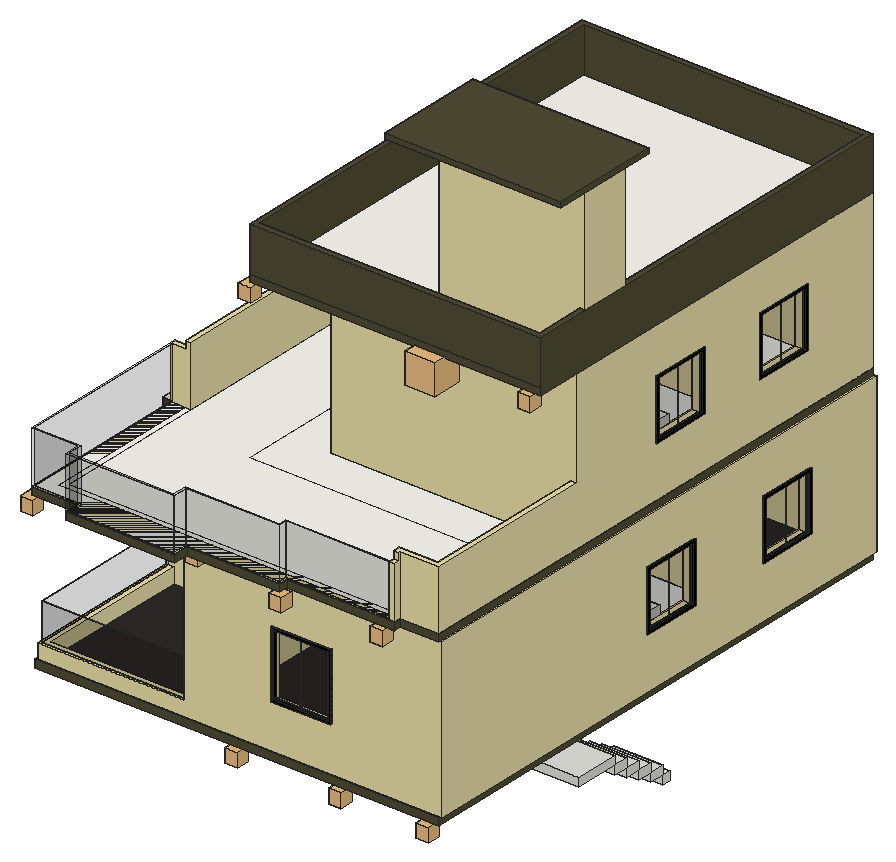
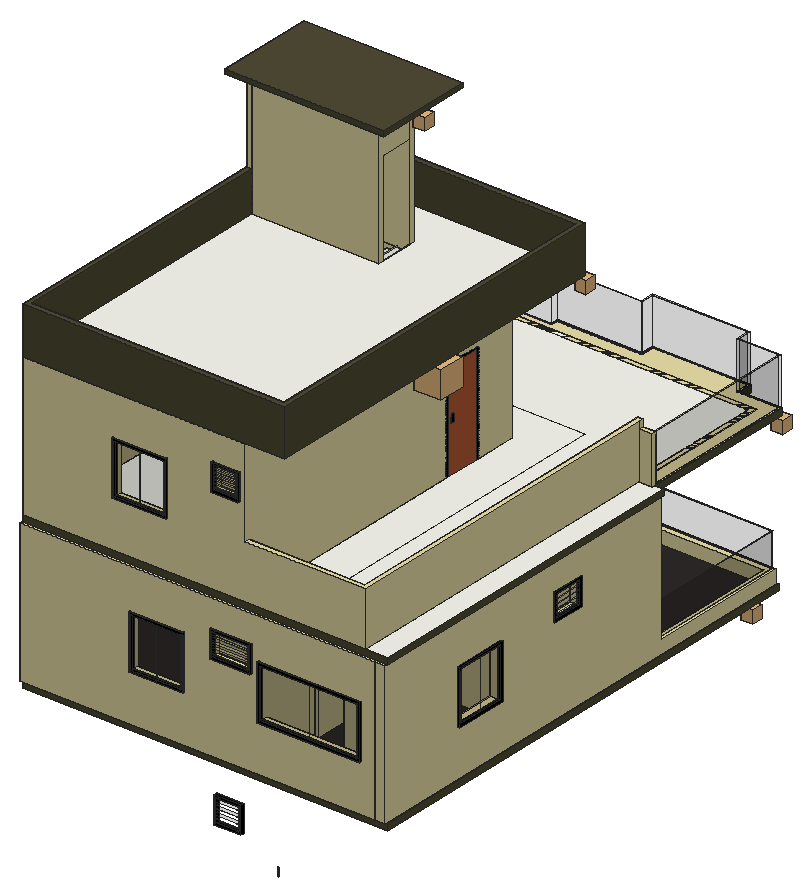
# SketchUp Ruby script. Lengths in inches.
U = 1.inch
M = Sketchup.active_model
def pt(a) = Geom::Point3d.new(a.map { |v| v * U })
def face(e, loops, mat)
  f = e.add_face(loops[0].map { |a| pt(a) })
  loops[1..].each { |l| e.add_face(l.map { |a| pt(a) }).erase! }
  f.material = f.back_material = mat if mat
  f
end
# faces: each face lists its corners as indices into pts; further lists are holes
def faces(e, pts, list, mat = nil) = list.each { |f| face(e, (f[0].is_a?(Array) ? f : [f]).map { |l| l.map { |i| pts[i] } }, mat) }
# xy, xz, yz: faces in a plane at the given z, y or x. An outline is a flat list of corners, or four numbers for a rectangle; further outlines are holes
def ring(l) = l.size == 4 ? [[l[0], l[1]], [l[2], l[1]], [l[2], l[3]], [l[0], l[3]]] : l.each_slice(2).to_a
def flat(e, list, mat, &to3) = list.each { |f| face(e, (f[0].is_a?(Array) ? f : [f]).map { |l| ring(l).map { |u, v| to3.(u, v) } }, mat) }
def xy(e, z, list, mat = nil) = flat(e, list, mat) { |x, y| [x, y, z] }
def xz(e, y, list, mat = nil) = flat(e, list, mat) { |x, z| [x, y, z] }
def yz(e, x, list, mat = nil) = flat(e, list, mat) { |y, z| [x, y, z] }
def lines(e, pts, list) = list.each { |a, b| e.add_line(pt(pts[a]), pt(pts[b])) }
# prism: a flat outline (further loops are holes) pulled along v
def prism(e, loops, v, mat = nil)
  f = face(e, loops, mat); d = Geom::Vector3d.new(v.map { |x| x * U })
  f.pushpull(f.normal.samedirection?(d) ? d.length : -d.length)
end
def box(e, o, s, mat = nil) = prism(e, [[o, [o[0] + s[0], o[1], o[2]], [o[0] + s[0], o[1] + s[1], o[2]], [o[0], o[1] + s[1], o[2]]]], [0, 0, s[2]], mat)
def at(x, y, z, deg = 0) = Geom::Transformation.translation(pt([x, y, z])) * Geom::Transformation.rotation(ORIGIN, Z_AXIS, deg.degrees)
def axes(o, x, y, z) = Geom::Transformation.new([*x, 0, *y, 0, *z, 0, *pt(o).to_a, 1])
def part(name) = M.definitions.add(name)
# library, detail: a bought-in or finely detailed component or shape, given as its bounding box
def library(name, o, s) = part(name).tap { |d| box(d.entities, o, s) }
def detail(e, o, s) = box(e.add_group.entities, o, s)
def put(e, d, t, mat = nil) = e.add_instance(d, t).tap { |i| i.material = mat if mat }
def group(e, t, mat = nil) = e.add_group.tap { |g| g.transformation = t; g.material = mat if mat }.entities
root = M.entities
M.materials.add("BLack FLOOR").color = [47, 42, 42]
M.materials.add("METAL").color = [0, 0, 0]
M.materials.add("WALL PAINT").color = [235, 224, 170]
M.materials.add("WALL PAINT\#1").color = [80, 76, 53]
M.materials.add("WHITE FLOOR").color = [250, 250, 243]
M.materials.add("glass").color = [0, 0, 0]
M.materials["glass"].alpha = 0.1
M.materials.add("wood").color = [181, 91, 54]
c1 = part("Component\#8")
box(c1.entities,[4.875,0,0],[7.125,36,7])
c2 = part("Stair tread")
box(c2.entities,[0,0,0],[12,39.4375,7])
c3 = library("Omni Light\#4",[-12,-12,-12],[24,24,24])
c4 = part("Stair landing \#4")
box(c4.entities,[-1.5,0,0],[36,39.4375,7])
c5 = part("Stair tread \#5")
box(c5.entities,[0,0,0],[12,39.4375,7])
c6 = library("Omni Light",[-12,-12,-12],[24,24,24])
c7 = library("Spot Light\#4",[-5.1,-5.1,-11.05],[10.2,10.2,11.05])
c8 = library("Spot Light\#5",[-5.1,-5.1,-11.05],[10.2,10.2,11.05])
c9 = library("Spot Light\#6",[-5.1,-5.1,-11.05],[10.2,10.2,11.05])
c10 = library("Spot Light\#7",[-5.1,-5.1,-11.05],[10.2,10.2,11.05])
c11 = library("Spot Light\#3",[-5.1,-5.1,-11.05],[10.2,10.2,11.05])
c12 = part("Stair tread \#1")
box(c12.entities,[-3.4375,0,0],[12,39.4375,7])
c13 = part("Stair landing")
box(c13.entities,[0,0,0],[39.4375,36,7])
c14 = part("Stair landing \#1")
box(c14.entities,[-1.5,0,0],[36,39.4375,7])
c15 = part("Stair tread \#3")
box(c15.entities,[-3.4375,0,0],[12,34.5,7])
c16 = part("Group173\#1")
p = [[0,0,0],[0,0,-9.21],[-2.27,0,-9.21],[14.78,-15.03,0],[-14.78,-15.03,0],[14.78,15.03,0],
  [14.78,0,0],[-14.78,15.03,0],[2.27,0,-9.21],[-14.78,0,0],[0,0,-14.91]]
lines(c16.entities,p,[[0,1],[1,2],[3,4],[5,6],[7,5],[1,8],[9,0],[0,6],[8,10],[4,9],[6,3],[2,10],
  [9,7]])
c17 = part("Rectangle Light")
put(c17.entities,c16,at(0,0,0))
c18 = library("Omni Light\#5",[-12,-12,-12],[24,24,24])
c19 = library("Omni Light\#1",[-12,-12,-12],[24,24,24])
c20 = library("Spot Light",[-5.1,-5.1,-11.05],[10.2,10.2,11.05])
c21 = library("Spot Light\#1",[-5.1,-5.1,-11.05],[10.2,10.2,11.05])
c22 = library("Spot Light\#2",[-5.1,-5.1,-11.05],[10.2,10.2,11.05])
c23 = library("Spot Light\#8",[-5.1,-5.1,-11.05],[10.2,10.2,11.05])
c24 = part("Stair tread \#2")
box(c24.entities,[0,0,0],[12,36,7])
c25 = part("Stair landing \#2")
box(c25.entities,[0,0,0],[36,36,7])
c26 = part("Stair landing \#3")
box(c26.entities,[-22.1875,0,0],[34.1875,36,7])
c27 = part("Stair tread \#4")
box(c27.entities,[-22.1875,0,0],[34.1875,12,7])
c28 = library("Omni Light\#2",[-12,-12,-12],[24,24,24])
c29 = library("Omni Light\#3",[-12,-12,-12],[24,24,24])
c30 = library("Spot Light\#9",[-5.1,-5.1,-11.05],[10.2,10.2,11.05])
c31 = library("Spot Light\#10",[-5.1,-5.1,-11.05],[10.2,10.2,11.05])
c32 = library("Spot Light\#11",[-5.1,-5.1,-11.05],[10.2,10.2,11.05])
put(root,c1,at(288,397.9,54.4375,-90))
g1 = group(root,at(112.46,576,55.32),"METAL")
box(g1,[0,0,0],[1.1,0.5,6.84])
put(root,c2,at(284.5625,385.9,61.4375,-90))
put(root,c2,at(284.5625,373.9,68.4375,-90))
put(root,c2,at(284.5625,361.9,75.4375,-90))
put(root,c3,at(252,402,93.375))
put(root,c2,at(284.5625,349.9,82.4375,-90))
g2 = group(root,at(138,585,83.4375))
prism(g2,[[[24,-1.5,24],[0,-1.5,24],[0,-1.5,0],[24,-1.5,0]],[[22,-1.5,22],[22,-1.5,2],[2,-1.5,2],[2,-1.5,22]]],[0,3,0],"METAL")
g3 = group(root,at(140,586.5,85.4375))
box(g3,[0,0,0],[20,0.2,3.53],"glass")
put(root,c4,at(284.5625,336.4,89.4375,-90))
g4 = group(root,at(140,586.5,90.93))
box(g4,[0,0,0],[20,0.2,3.53],"glass")
g5 = group(root,at(140,586.5,96.42))
box(g5,[0,0,0],[20,0.2,3.53],"glass")
g6 = group(root,at(224.5625,301.9,89.4375))
put(g6,c5,at(0,0,35))
put(g6,c2,at(48,0,7))
put(g6,c2,at(36,0,14))
put(g6,c2,at(12,0,28))
put(g6,c2,at(24,0,21))
g7 = group(root,at(140,586.5,101.91))
box(g7,[0,0,0],[20,0.2,3.53],"glass")
put(root,c6,at(106.39,205.09,117.1875))
put(root,c7,at(93.68,171.67,131.43))
put(root,c8,at(171,150,131.43))
put(root,c9,at(253.9375,150,131.43))
put(root,c10,at(324.18,150,131.43))
put(root,c11,at(10.5,179.06,132.58))
g8 = group(root,at(32,150,131.4375),"WALL PAINT\#1")
xy(g8,0,[[[-23,0,301,435],[192.5625,151.1875,292,271.5]]],"WALL PAINT\#1")
xy(g8,6,[[[-23,0,301,435],[192.5625,151.1875,292,271.5]]],"BLack FLOOR")
xz(g8,0,[[-23,0,301,6]],"WALL PAINT\#1")
xz(g8,151.1875,[[192.5625,0,292,6]],"WALL PAINT\#1")
xz(g8,271.5,[[192.5625,0,292,6]],"WALL PAINT\#1")
xz(g8,435,[[-23,0,301,6]],"WALL PAINT\#1")
yz(g8,-23,[[0,0,435,6]],"WALL PAINT\#1")
yz(g8,192.5625,[[151.1875,0,271.5,6]],"WALL PAINT\#1")
yz(g8,292,[[151.1875,0,271.5,6]],"WALL PAINT\#1")
yz(g8,301,[[0,0,435,6]],"WALL PAINT\#1")
g9 = group(root,at(9,150,137.4375))
put(g9,c12,at(256.5,230.5,21))
put(g9,c12,at(277.0625,215.0625,49,-90))
put(g9,c12,at(232.5,230.5,7))
put(g9,c12,at(244.5,230.5,14))
put(g9,c13,at(277.0625,230.5,35))
put(g9,c12,at(277.0625,191.0625,63,-90))
put(g9,c12,at(277.0625,179.0625,70,-90))
put(g9,c12,at(220.5,230.5,0))
put(g9,c12,at(268.5,230.5,28))
put(g9,c14,at(277.0625,169,77,-90))
put(g9,c12,at(277.0625,227.0625,42,-90))
put(g9,c15,at(268.5,136,84))
put(g9,c12,at(277.0625,203.0625,56,-90))
put(g9,c15,at(256.5,136,91))
put(g9,c15,at(244.5,136,98))
put(g9,c15,at(232.5,136,105))
put(g9,c15,at(220.5,136,112))
put(g9,c15,at(208.5,136,119))
put(g9,c17,axes([157,118.76,110.97],[-0.60781,0.79408,0],[0,0,-1],[0.79408,0.60781,0]))
put(g9,c18,at(205.65,130.5,40.02))
g10 = group(g9,at(325.4375,324.24,44))
box(g10,[-0.31,0,0],[0.31,22,44],"glass")
g11 = group(g9,at(68,436.25,44))
box(g11,[0,-0.31,0],[43.5,0.31,44],"glass")
g12 = group(g9,at(24.5,436.56,44))
box(g12,[0,-0.31,0],[43.5,0.31,44],"glass")
g13 = group(g9,at(0,220.96,96.53))
yz(g13,0,[[0,0,26,3.47]],"glass")
g14 = group(g9,at(-10.5,-10.5,0),"WALL PAINT")
xy(g14,0,[[12,12,12,447,21,447,21,140.5,18,140.5,18,18,129,18,129,140.5,81,140.5,81,146.5,135,146.5,135,19,327,19,327,69,309,69,309,74.5,327,74.5,327,141,279,141,279,69,273.5,69,273.5,141,177,141,177,146.5,327,146.5,327,438,184,438,184,378.42,178,378.42,178,438,130,438,130,283,178,283,178,342.42,184,342.42,184,277,124,277,124,438,33,438,33,447,336,447,336,12],[94,277,96,279],[122,277,124,279]])
xy(g14,12,[[12,12,129,12,129,13.5625,14.02,13.5625,14.02,140.5,12,140.5],[14.33,13.88,129,13.88,129,18,18,18,18,140.5,14.33,140.5]])
xy(g14,36,[[199.7,12,247.7,19]])
xy(g14,42,[[14.02,13.5625,129,13.5625,129,13.88,14.33,13.88,14.33,140.5,14.02,140.5],[327,216.47,336,264.47],[12,318.73,21,366.73],[327,332.74,336,380.74],[33,438,124,447],
  [190,438,238,447]])
xy(g14,78,[[12,229.46,21,259.46],[130,438,166,447]])
xy(g14,88,[[96,277,122,279]])
xy(g14,90,[[199.7,12,247.7,19],[279,69,309,74.5],[33,140.5,81,146.5],[135,141,177,146.5],[69,205,73.5,235],
  [327,216.47,336,264.47],[94,277,124,279],[184,277,220,283],[94,279,124,283],[12,318.73,21,366.73],
  [327,332.74,336,380.74],[178,342.42,184,378.42],[94,384,124,390],[33,438,124,447],[190,438,238,447]])
xy(g14,102,[[12,229.46,21,259.46],[130,438,166,447]])
xy(g14,126,[[[129,12,336,12,336,447,21,447,21,438,124,438,124,390,21,390,21,447,12,447,12,140.5,129,140.5],[21,146.5,21,200.5,73.5,200.5,73.5,277,327,277,327,146.5],[184,283,327,438],[135,19,135,141,273.5,141,273.5,69,327,69,327,19],[21,283,124,384],[130,283,178,438],[21,205,69,277],[279,74.5,327,141]]])
xz(g14,12,[[[12,0,336,0,336,126,129,126,129,12,12,12],[199.7,36,247.7,90]]])
xz(g14,13.5625,[[14.02,12,129,42]],"glass")
xz(g14,13.88,[[14.33,12,129,42]],"glass")
xz(g14,18,[[18,0,129,12]])
xz(g14,19,[[[135,0,327,126],[199.7,36,247.7,90]]])
xz(g14,69,[[273.5,0,279,0,279,90,309,90,309,0,327,0,327,126,273.5,126]])
xz(g14,74.5,[[309,0,309,90,279,90,279,126,327,126,327,0]])
xz(g14,140.5,[[18,0,33,0,33,90,81,90,81,0,129,0,129,126,12,126,12,12,14.02,12,14.02,42,14.33,42,14.33,12,18,12]])
xz(g14,141,[[177,0,273.5,0,273.5,126,135,126,135,90,177,90],[279,0,327,126]])
xz(g14,146.5,[[21,0,21,126,327,126,327,0,177,0,177,90,135,90,135,0,81,0,81,90,33,90,33,0]])
xz(g14,200.5,[[21,0,73.5,126]],"WHITE FLOOR")
xz(g14,205,[[21,0,21,126,69,126,69,90,73.5,90,73.5,0]])
xz(g14,216.47,[[327,42,336,90]])
xz(g14,229.46,[[12,78,21,102]])
xz(g14,235,[[69,0,73.5,90]])
xz(g14,259.46,[[12,78,21,102]])
xz(g14,264.47,[[327,42,336,90]])
xz(g14,277,[[21,0,69,126],[73.5,0,94,0,94,90,124,90,124,0,184,0,184,90,220,90,220,0,327,0,327,126,73.5,126],[94,0,96,0,96,88,122,88,122,0,124,0,124,90,94,90]])
xz(g14,279,[[94,0,94,90,124,90,124,0,122,0,122,88,96,88,96,0]])
xz(g14,283,[[21,0,21,126,124,126,124,90,94,90,94,0],[130,0,178,126],[220,0,220,90,184,90,184,126,327,126,327,0]])
xz(g14,318.73,[[12,42,21,90]])
xz(g14,332.74,[[327,42,336,90]])
xz(g14,342.42,[[178,0,184,90]])
xz(g14,366.73,[[12,42,21,90]])
xz(g14,378.42,[[178,0,184,90]])
xz(g14,380.74,[[327,42,336,90]])
xz(g14,384,[[21,0,94,0,94,90,124,90,124,126,21,126]])
xz(g14,390,[[21,0,21,126,124,126,124,90,94,90,94,0]])
xz(g14,438,[[21,0,124,0,124,42,33,42,33,90,124,90,124,126,21,126],[130,0,178,0,178,126,130,126,130,102,166,102,166,78,130,78],[[184,0,327,126],[190,42,238,90]]])
xz(g14,447,[[12,0,21,126],[[21,0,336,126],[33,42,124,90],[190,42,238,90],[130,78,166,102]]])
yz(g14,12,[[[12,0,12,12,140.5,12,140.5,126,447,126,447,0],[318.73,42,366.73,90],[229.46,78,259.46,102]]])
yz(g14,14.02,[[13.5625,12,140.5,42]],"glass")
yz(g14,14.33,[[13.88,12,140.5,42]],"glass")
yz(g14,18,[[18,0,140.5,12]])
yz(g14,21,[[146.5,0,200.5,126],[[205,0,277,126],[229.46,78,259.46,102]],[[283,0,384,126],[318.73,42,366.73,90]],[390,0,438,126],[438,0,447,126]])
yz(g14,33,[[140.5,0,146.5,90],[438,42,447,90]])
yz(g14,69,[[235,0,235,90,205,90,205,126,277,126,277,0]])
yz(g14,73.5,[[200.5,0,205,0,205,90,235,90,235,0,277,0,277,126,200.5,126]])
yz(g14,81,[[140.5,0,146.5,90]])
yz(g14,94,[[277,0,279,90],[279,0,283,90],[384,0,390,90]])
yz(g14,96,[[277,0,279,88]])
yz(g14,122,[[277,0,279,88]])
yz(g14,124,[[277,0,279,90],[279,0,279,90,283,90,283,126,384,126,384,0],[384,0,384,90,390,90,390,126,438,126,438,90,447,90,447,42,438,42,438,0]])
yz(g14,129,[[18,0,18,12,13.88,12,13.88,42,13.5625,42,13.5625,12,12,12,12,126,140.5,126,140.5,0]])
yz(g14,130,[[283,0,438,0,438,78,447,78,447,102,438,102,438,126,283,126]])
yz(g14,135,[[19,0,146.5,0,146.5,90,141,90,141,126,19,126]])
yz(g14,166,[[438,78,447,102]])
yz(g14,177,[[141,0,146.5,90]])
yz(g14,178,[[283,0,283,126,438,126,438,0,378.42,0,378.42,90,342.42,90,342.42,0]])
yz(g14,184,[[277,0,342.42,0,342.42,90,378.42,90,378.42,0,438,0,438,126,283,126,283,90,277,90]])
yz(g14,190,[[438,42,447,90]])
yz(g14,199.7,[[12,36,19,90]])
yz(g14,220,[[277,0,283,90]])
yz(g14,238,[[438,42,447,90]])
yz(g14,247.7,[[12,36,19,90]])
yz(g14,273.5,[[69,0,141,126]])
yz(g14,279,[[69,0,141,0,141,126,74.5,126,74.5,90,69,90]])
yz(g14,309,[[69,0,74.5,90]])
yz(g14,327,[[19,0,69,126],[74.5,0,141,126],[[146.5,0,277,126],[216.47,42,264.47,90]],[[283,0,438,126],[332.74,42,380.74,90]]])
yz(g14,336,[[[12,0,447,126],[332.74,42,380.74,90],[216.47,42,264.47,90]]])
p = [[184,342.42,0],[184,378.42,0]]
lines(g14,p,[[0,1]])
g15 = group(g14,at(279,69,0))
prism(g15,[[[2,2,0],[0,2,0],[0,2,90],[30,2,90],[30,2,0],[28,2,0],[28,2,88],[2,2,88]]],[0,-2,0])
g16 = group(g14,at(73.5,205,0))
prism(g16,[[[0,0,0],[0,2,0],[0,2,88],[0,28,88],[0,28,0],[0,30,0],[0,30,90],[0,0,90]]],[-2,0,0])
g17 = group(g14,at(184,277,0))
prism(g17,[[[0,0,0],[2,0,0],[2,0,88],[34,0,88],[34,0,0],[36,0,0],[36,0,90],[0,0,90]]],[0,2,0])
g18 = group(g14,at(184,342.42,0))
prism(g18,[[[0,36,0],[0,36,90],[0,0,90],[0,0,0]],[[0,34,2],[0,2,2],[0,2,88],[0,34,88]]],[-2,0,0])
g19 = group(g14,at(94,384,0))
prism(g19,[[[0,0,0],[2,0,0],[2,0,88],[28,0,88],[28,0,0],[30,0,0],[30,0,90],[0,0,90]]],[0,2,0])
g20 = group(g9,at(189.2,1.5,36),"METAL")
prism(g20,[[[48,1.5,54],[48,1.5,0],[0,1.5,0],[0,1.5,54]],[[2,1.5,2],[46,1.5,2],[46,1.5,52],[2,1.5,52]]],[0,-3,0])
g21 = group(g9,at(121.5,438,88.59))
box(g21,[0,-0.2,0],[32,0.2,2.82],"glass")
g22 = group(g9,at(121.5,438,84.29))
box(g22,[0,-0.2,0],[32,0.2,2.82],"glass")
g23 = group(g9,at(121.5,438,80))
box(g23,[0,-0.2,0],[32,0.2,2.82],"glass")
g24 = group(g9,at(22.5,436.5,42))
prism(g24,[[[91,1.5,0],[0,1.5,0],[0,1.5,48],[91,1.5,48]],[[89,1.5,46],[2,1.5,46],[2,1.5,2],[89,1.5,2]]],[0,-3,0],"METAL")
g25 = group(g9,at(121.5,438,92.88))
box(g25,[0,-0.2,0],[32,0.2,2.82],"glass")
g26 = group(g9,at(119.5,436.5,78))
prism(g26,[[[0,-1.5,0],[36,-1.5,0],[36,-1.5,24],[0,-1.5,24]],[[2,-1.5,22],[34,-1.5,22],[34,-1.5,2],[2,-1.5,2]]],[0,3,0],"METAL")
g27 = group(g9,at(121.5,438,97.18))
box(g27,[0,-0.2,0],[32,0.2,2.82],"glass")
g28 = group(g9,at(179.5,436.5,42))
prism(g28,[[[48,-1.5,0],[48,-1.5,48],[0,-1.5,48],[0,-1.5,0]],[[2,-1.5,46],[46,-1.5,46],[46,-1.5,2],[2,-1.5,2]]],[0,3,0],"METAL")
g29 = group(g9,at(325.5,205.97,42))
xy(g29,0,[[-1.5,0,1.5,48]],"METAL")
xy(g29,2,[[-1.5,2,1.5,46]],"METAL")
xy(g29,46,[[-1.5,2,1.5,46]],"METAL")
xy(g29,48,[[-1.5,0,1.5,48]],"METAL")
xz(g29,0,[[-1.5,0,1.5,48]],"METAL")
xz(g29,2,[[-1.5,2,1.5,46]],"METAL")
xz(g29,46,[[-1.5,2,1.5,46]],"METAL")
xz(g29,48,[[-1.5,0,1.5,48]],"METAL")
yz(g29,-1.5,[[[0,0,48,48],[2,2,46,46]]],"METAL")
yz(g29,1.5,[[[0,0,48,48],[2,2,46,46]]],"METAL")
g30 = group(g29,at(-0.4375,2,2))
box(g30,[-0.31,0,0],[0.31,22,44],"glass")
g31 = group(g29,at(-0.12,24,2))
box(g31,[-0.31,0,0],[0.31,22,44],"glass")
g32 = group(g9,at(191.2,0.68,38.89))
box(g32,[0,0,0],[22,0.31,50],"glass")
g33 = group(g9,at(213.2,1,38))
box(g33,[0,0,0],[22,0.31,50],"glass")
g34 = group(g9,at(325.5,322.24,42))
prism(g34,[[[-1.5,48,48],[-1.5,48,0],[-1.5,0,0],[-1.5,0,48]],[[-1.5,2,46],[-1.5,2,2],[-1.5,46,2],[-1.5,46,46]]],[3,0,0],"METAL")
g35 = group(g9,at(325.75,346.24,44))
box(g35,[-0.31,0,0],[0.31,22,44],"glass")
g36 = group(g9,at(0,220.96,92.4))
yz(g36,0,[[0,0,26,3.47]],"glass")
g37 = group(g9,at(0,220.96,88.26))
yz(g37,0,[[0,0,26,3.47]],"glass")
g38 = group(g9,at(0,220.96,80))
yz(g38,0,[[0,0,26,3.47]],"glass")
g39 = group(g9,at(0,220.96,84.13))
yz(g39,0,[[0,0,26,3.47]],"glass")
g40 = group(g9,at(1.5,218.96,78))
prism(g40,[[[1.5,0,0],[1.5,30,0],[1.5,30,24],[1.5,0,24]],[[1.5,2,2],[1.5,2,22],[1.5,28,22],[1.5,28,2]]],[-3,0,0],"METAL")
g41 = group(g9,at(181.5,436.5,44))
box(g41,[0,-0.31,0],[22,0.31,44],"glass")
g42 = group(g9,at(203.5,436.1875,44))
box(g42,[0,-0.31,0],[22,0.31,44],"glass")
g43 = group(g9,at(124.5,136,0))
prism(g43,[[[42,0,0],[40,0,0],[40,0,88],[2,0,88],[2,0,0],[0,0,0],[0,0,90],[42,0,90]]],[0,-2,0])
g44 = group(g9,at(22.5,130,0))
prism(g44,[[[0,0,0],[2,0,0],[2,0,88],[46,0,88],[46,0,0],[48,0,0],[48,0,90],[0,0,90]]],[0,2,0],"METAL")
g45 = group(g9,at(-1.0625,332.4,44))
box(g45,[0,0,0],[0.31,22,44],"glass")
g46 = group(g9,at(-1.0625,310.4,44))
box(g46,[0,0,0],[0.31,22,44],"glass")
g47 = group(g9,at(0.4375,308.4,42))
prism(g47,[[[1.5,48,48],[1.5,0,48],[1.5,0,0],[1.5,48,0]],[[1.5,2,46],[1.5,46,46],[1.5,46,2],[1.5,2,2]]],[-3,0,0],"METAL")
g48 = group(root,at(33.5,280,137.4375),"wood")
box(g48,[0,0,0],[44,0.71,88])
g49 = group(root,at(38.99,280,184.9375),"METAL")
box(g49,[0,-0.5625,0],[1.25,0.5625,5.25])
put(root,c19,at(70,223.72,250.3125))
put(root,c20,at(137.83,151.5,263.43))
put(root,c21,at(215.4,138,263.43))
put(root,c22,at(291.81,144.43,263.43))
put(root,c23,at(16.5,138,263.43))
g50 = group(root,at(32,150,263.4375),"WALL PAINT")
xy(g50,0,[[[21.6,-24,21.6,-12,-15.5,-12,-15.5,128.5625,-23,128.5625,-23,435,301,435,301,0,270.2,0,270.2,-5.57,183.4,-5.57,183.4,-12,108.4,-12,108.4,-24],[192.5625,151.1875,292,271.5]]],"WALL PAINT\#1")
xy(g50,6,[[[21.6,-24,108.4,-24,108.4,-12,183.4,-12,183.4,-5.57,270.2,-5.57,270.2,0,301,0,301,435,-23,435,-23,128.5625,-15.5,128.5625,-15.5,-12,21.6,-12],[192.5625,151.1875,292,271.5]]],"WHITE FLOOR")
xz(g50,-24,[[21.6,0,108.4,6]],"WALL PAINT\#1")
xz(g50,-12,[[-15.5,0,21.6,6],[108.4,0,183.4,6]],"WALL PAINT\#1")
xz(g50,-5.57,[[183.4,0,270.2,6]],"WALL PAINT\#1")
xz(g50,0,[[270.2,0,301,6]],"WALL PAINT\#1")
xz(g50,128.5625,[[-23,0,-15.5,6]],"WALL PAINT\#1")
xz(g50,151.1875,[[192.5625,0,292,6]],"WALL PAINT\#1")
xz(g50,271.5,[[192.5625,0,292,6]],"WALL PAINT\#1")
xz(g50,435,[[-23,0,301,6]],"WALL PAINT\#1")
yz(g50,-23,[[128.5625,0,435,6]],"WALL PAINT\#1")
yz(g50,-15.5,[[-12,0,128.5625,6]],"WALL PAINT\#1")
yz(g50,21.6,[[-24,0,-12,6]],"WALL PAINT\#1")
yz(g50,108.4,[[-24,0,-12,6]],"WALL PAINT\#1")
yz(g50,183.4,[[-12,0,-5.57,6]],"WALL PAINT\#1")
yz(g50,192.5625,[[151.1875,0,271.5,6]],"WALL PAINT\#1")
yz(g50,270.2,[[-5.57,0,0,6]],"WALL PAINT\#1")
yz(g50,292,[[151.1875,0,271.5,6]],"WALL PAINT\#1")
yz(g50,301,[[0,0,435,6]],"WALL PAINT\#1")
g51 = group(root,at(16.5,126,269.4375))
xy(g51,0,[[37.1,0,37.1,12,0,12,0,155.5,12,155.5,12,459,236.5,459,236.5,450,176.5,450,176.5,400.55,172,400.55,172,450,124,450,124,306,172,306,172,370.55,176.5,370.55,176.5,301.5,124,301.5,124,235.28,119.5,235.28,119.5,454.5,16.5,454.5,16.5,151,1.5,151,1.5,13.5,38.6,13.5,38.6,1.5,122.4,1.5,122.4,13.5,197.4,13.5,197.4,19.93,281.2,19.93,281.2,18.43,198.9,18.43,198.9,12,123.9,12,123.9,0],[38.6,1.5,38.6,13.5,1.5,13.5,1.5,151,12,151,12,24,281.2,24,281.2,19.93,197.4,19.93,197.4,13.5,122.4,13.5,122.4,1.5],[281.27,18.43,281.27,22.93,281.2,22.93,281.2,28.5,312,28.5,312,162,119.5,162,119.5,199.28,124,199.28,124,171,307.5,171,307.5,288.97,316.5,288.97,316.5,24,285.7,24,285.7,18.43],[281.2,18.43,281.27,22.93],[12,24,281.2,24,281.2,28.5,16.5,28.5,16.5,151,12,151],
  [307.5,344.19,316.5,392.19]],"WALL PAINT")
xy(g51,42,[[281.2,18.43,285.7,22.93],[0,151,12,155.5],[307.5,240.97,316.5,288.97],[307.5,344.19,316.5,392.19],[188.5,450,236.5,459]],"WALL PAINT")
xy(g51,42,[[37.1,0,123.9,0,123.9,12,198.9,12,198.9,18.43,281.2,18.43,281.2,19.93,197.4,19.93,197.4,13.5,122.4,13.5,122.4,1.5,38.6,1.5,38.6,13.5,1.5,13.5,1.5,151,0,151,0,12,37.1,12]],"glass")
xy(g51,48,[[281.2,22.93,285.7,22.93,285.7,24,316.5,24,316.5,162,312,162,312,28.5,281.2,28.5],[12,151,16.5,151,16.5,454.5,119.5,454.5,119.5,459,12,459]],"WALL PAINT")
xy(g51,78,[[124,450,148,459]],"WALL PAINT")
xy(g51,90,[[119.5,199.28,124,235.28],[307.5,240.97,316.5,288.97],[176.5,301.5,206.78,306],[307.5,344.19,316.5,392.19],[172,370.55,176.5,400.55],
  [188.5,450,236.5,459]],"WALL PAINT")
xy(g51,102,[[124,450,148,459]],"WALL PAINT")
xy(g51,126,[[[119.5,162,316.5,459],[124,171,307.5,301.5],[176.5,306,307.5,450],[124,306,172,450]]],"WALL PAINT")
xz(g51,0,[[37.1,0,123.9,42]],"glass")
xz(g51,1.5,[[38.6,0,122.4,42]],"glass")
xz(g51,12,[[0,0,37.1,42],[123.9,0,198.9,42]],"glass")
xz(g51,13.5,[[1.5,0,38.6,42],[122.4,0,197.4,42]],"glass")
xz(g51,18.43,[[281.2,0,285.7,42]],"WALL PAINT")
xz(g51,18.43,[[198.9,0,281.2,42]],"glass")
xz(g51,19.93,[[197.4,0,281.2,42]],"glass")
xz(g51,22.93,[[281.2,0,281.27,42],[281.2,42,285.7,48]],"WALL PAINT")
xz(g51,24,[[285.7,0,316.5,48]],"WALL PAINT")
xz(g51,28.5,[[281.2,0,312,48]],"WALL PAINT")
xz(g51,151,[[1.5,0,16.5,0,16.5,48,12,48,12,42,1.5,42]],"WALL PAINT")
xz(g51,155.5,[[0,0,12,42]],"WALL PAINT")
xz(g51,162,[[119.5,0,312,0,312,48,316.5,48,316.5,126,119.5,126]],"WALL PAINT")
xz(g51,171,[[124,0,307.5,126]],"WALL PAINT")
xz(g51,199.28,[[119.5,0,124,90]],"WALL PAINT")
xz(g51,235.28,[[119.5,0,124,90]],"WALL PAINT")
xz(g51,240.97,[[307.5,42,316.5,90]],"WALL PAINT")
xz(g51,288.97,[[307.5,42,316.5,90]],"WALL PAINT")
xz(g51,301.5,[[124,0,176.5,0,176.5,90,206.78,90,206.78,0,307.5,0,307.5,126,124,126]],"WALL PAINT")
xz(g51,306,[[124,0,172,126],[206.78,0,206.78,90,176.5,90,176.5,126,307.5,126,307.5,0]],"WALL PAINT")
xz(g51,344.19,[[307.5,42,316.5,90]],"WALL PAINT")
xz(g51,370.55,[[172,0,176.5,90]],"WALL PAINT")
xz(g51,392.19,[[307.5,42,316.5,90]],"WALL PAINT")
xz(g51,400.55,[[172,0,176.5,90]],"WALL PAINT")
xz(g51,450,[[124,0,172,0,172,126,124,126,124,102,148,102,148,78,124,78],[[176.5,0,307.5,126],[188.5,42,236.5,90]]],"WALL PAINT")
xz(g51,454.5,[[16.5,0,119.5,48]],"WALL PAINT")
xz(g51,459,[[[12,0,12,48,119.5,48,119.5,126,316.5,126,316.5,0],[188.5,42,236.5,90],[124,78,148,102]]],"WALL PAINT")
yz(g51,0,[[151,0,155.5,42]],"WALL PAINT")
yz(g51,0,[[12,0,151,42]],"glass")
yz(g51,1.5,[[13.5,0,151,42]],"glass")
yz(g51,12,[[155.5,0,459,48],[151,42,155.5,48]],"WALL PAINT")
yz(g51,16.5,[[151,0,454.5,48]],"WALL PAINT")
yz(g51,37.1,[[0,0,12,42]],"glass")
yz(g51,38.6,[[1.5,0,13.5,42]],"glass")
yz(g51,119.5,[[162,0,162,126,459,126,459,48,454.5,48,454.5,0,235.28,0,235.28,90,199.28,90,199.28,0]],"WALL PAINT")
yz(g51,122.4,[[1.5,0,13.5,42]],"glass")
yz(g51,123.9,[[0,0,12,42]],"glass")
yz(g51,124,[[171,0,199.28,0,199.28,90,235.28,90,235.28,0,301.5,0,301.5,126,171,126],[306,0,450,0,450,78,459,78,459,102,450,102,450,126,306,126]],"WALL PAINT")
yz(g51,148,[[450,78,459,102]],"WALL PAINT")
yz(g51,172,[[306,0,306,126,450,126,450,0,400.55,0,400.55,90,370.55,90,370.55,0]],"WALL PAINT")
yz(g51,176.5,[[301.5,0,370.55,0,370.55,90,400.55,90,400.55,0,450,0,450,126,306,126,306,90,301.5,90]],"WALL PAINT")
yz(g51,188.5,[[450,42,459,90]],"WALL PAINT")
yz(g51,197.4,[[13.5,0,19.93,42]],"glass")
yz(g51,198.9,[[12,0,18.43,42]],"glass")
yz(g51,206.78,[[301.5,0,306,90]],"WALL PAINT")
yz(g51,236.5,[[450,42,459,90]],"WALL PAINT")
yz(g51,281.2,[[18.43,0,19.93,42]])
yz(g51,281.2,[[19.93,0,22.93,42],[22.93,0,28.5,48]],"WALL PAINT")
yz(g51,285.7,[[18.43,0,24,0,24,48,22.93,48,22.93,42,18.43,42]],"WALL PAINT")
yz(g51,307.5,[[[171,0,301.5,126],[240.97,42,288.97,90]],[[306,0,450,126],[344.19,42,392.19,90]]],"WALL PAINT")
yz(g51,312,[[28.5,0,162,48]],"WALL PAINT")
yz(g51,316.5,[[[24,0,459,0,459,126,162,126,162,48,24,48],[344.19,42,392.19,90],[240.97,42,288.97,90]]],"WALL PAINT")
g52 = group(g51,at(315.9375,346.19,44))
box(g52,[-0.31,0,0],[0.31,22,44],"glass")
g53 = group(g51,at(126,460.5,97.9))
box(g53,[0,-0.2,0],[20,0.2,2.1],"glass")
g54 = group(g51,at(124,459,78))
prism(g54,[[[24,1.5,0],[0,1.5,0],[0,1.5,24],[24,1.5,24]],[[2,1.5,2],[22,1.5,2],[22,1.5,22],[2,1.5,22]]],[0,-3,0],"METAL")
g55 = group(g51,at(119.5,199.28,0),"METAL")
prism(g55,[[[0,36,0],[0,34,0],[0,34,88],[0,2,88],[0,2,0],[0,0,0],[0,0,90],[0,36,90]]],[2,0,0])
g56 = group(g51,at(176.5,301.5,0))
prism(g56,[[[0,0,0],[2,0,0],[2,0,88],[28.28,0,88],[28.28,0,0],[30.28,0,0],[30.28,0,90],[0,0,90]]],[0,2,0])
g57 = group(g51,at(0,0,0))
g58 = group(g57,at(0,0,0))
xy(g58,0,[[307.5,288.97,316.5,288.97,316.5,344.19,307.5,344.19,307.5,306,206.78,306,206.78,301.5,307.5,301.5]])
p = [[307.5,240.97,0],[311,240.97,0],[0,24,0],[0,12,0],[259.5,171,0],[259.5,207,0],
  [119.5,459,0],[119.5,454.5,0],[312,392.19,0],[312,344.19,0],[16.5,454.5,0],[16.5,155.5,0],
  [271.5,265.5,0],[271.5,301.5,0],[307.5,237.22,0],[271.5,237.22,0],[313,288.97,0],[313,240.97,0],
  [316.5,459,0],[316.5,392.19,0],[316.5,24,0],[285.6,24,0],[307.5,217.07,0],[271.5,217.07,0],
  [307.5,392.19,0],[311,392.19,0],[211.5,171,0],[223.5,171,0],[313,392.19,0],[313,344.19,0],
  [16.5,28.5,0],[247.5,265.5,0],[247.5,301.5,0],[316.5,28.5,0],[12,459,0],[12,454.5,0],
  [307.5,450,0],[316.5,126,0],[119.5,126,0],[83.5,126,0],[83.5,454.5,0],[211.5,207,0],
  [235.5,171,0],[235.5,207,0],[247.5,171,0],[247.5,207,0],[235.5,265.5,0],[235.5,301.5,0],
  [307.5,227.15,0],[271.5,227.15,0],[307.5,247.29,0],[271.5,247.29,0],[223.5,207,0],[311,344.19,0],
  [312,288.97,0],[312,240.97,0],[236.5,450,0],[124,450,0],[124,306,0],[12,155.5,0],
  [0,155.5,0],[37.1,12,0],[37.1,0,0],[123.9,0,0],[311,288.97,0],[12,24,0],
  [123.9,12,0],[271.5,171,0],[271.5,207,0],[259.5,265.5,0],[259.5,301.5,0],[198.8,12,0],
  [271.5,257.37,0],[236.5,453.5,0],[188.5,450,0],[188.5,453.5,0],[211.5,162,0],[316.5,162,0],
  [172,306,0],[198.8,18.43,0],[285.6,18.43,0],[172,450,0],[172,400.55,0],[176.5,370.55,0],
  [172,370.55,0],[176.5,400.55,0],[176.5,301.5,0],[124,301.5,0],[148,454.5,0],[124,454.5,0],
  [223.5,265.5,0],[236.5,455.5,0],[188.5,455.5,0],[124,235.28,0],[148,459,0],[236.5,454.5,0],
  [188.5,454.5,0],[119.5,199.28,0],[119.5,162,0],[148,450,0],[176.5,450,0],[124,199.28,0],
  [124,171,0],[307.5,207,0],[236.5,459,0],[119.5,235.28,0],[124,459,0],[188.5,459,0],
  [307.5,344.19,0],[316.5,240.97,0],[316.5,155.5,0],[307.5,288.97,0],[307.5,265.5,0],[316.5,344.19,0],
  [307.5,257.37,0],[307.5,171,0],[12,307.25,0],[316.5,288.97,0],[316.5,119.5,0]]
lines(g58,p,[[0,1],[2,3],[4,5],[6,7],[8,9],[10,11],[12,13],[14,15],[16,17],[18,19],[20,21],[22,23],
  [24,25],[26,27],[28,29],[11,30],[31,32],[33,30],[34,35],[36,24],[37,38],[39,40],[26,41],[42,43],
  [44,45],[46,47],[48,49],[50,51],[41,52],[25,53],[34,6],[54,55],[36,56],[57,58],[59,60],[27,52],
  [60,2],[3,61],[61,62],[62,63],[64,1],[59,65],[35,10],[63,66],[67,68],[69,70],[66,71],[8,28],
  [72,51],[25,8],[56,73],[74,75],[76,77],[78,58],[79,80],[81,82],[83,84],[82,85],[86,87],[38,39],
  [88,89],[27,42],[90,46],[91,92],[23,68],[80,21],[87,93],[94,88],[71,79],[95,96],[97,98],[57,99],
  [100,85],[97,101],[101,102],[57,89],[83,86],[68,103],[84,78],[76,98],[26,102],[104,91],[52,43],[49,23],
  [93,105],[15,49],[51,15],[73,75],[55,17],[1,55],[6,106],[92,107],[4,67],[24,108],[50,0],[75,96],
  [7,105],[10,40],[109,77],[21,65],[89,106],[48,22],[110,37],[111,112],[46,31],[74,100],[40,7],[31,69],
  [19,113],[73,95],[42,44],[17,109],[45,5],[14,48],[114,50],[88,99],[77,110],[103,115],[28,19],[91,95],
  [44,4],[56,74],[116,59],[94,107],[117,109],[33,20],[35,116],[22,103],[106,94],[99,81],[0,14],[118,33],
  [43,45],[96,92],[37,118],[107,104],[67,115],[104,18],[69,12],[5,68],[114,72],[112,114],[12,112],[12,72]])
put(g58,c24,at(211.5,265.5,0))
put(g58,c24,at(223.5,265.5,7))
put(g58,c24,at(235.5,265.5,14))
put(g58,c24,at(247.5,265.5,21))
put(g58,c24,at(259.5,265.5,28))
put(g58,c25,at(271.5,265.5,35))
put(g58,c24,at(307.5,253.5,42,90))
put(g58,c24,at(307.5,241.5,49,90))
put(g58,c24,at(307.5,229.5,56,90))
put(g58,c24,at(307.5,217.5,63,90))
put(g58,c24,at(307.5,205.5,70,90))
put(g58,c26,at(307.5,193.5,77,90))
put(g58,c27,at(271.5,193.5,84,90))
put(g58,c27,at(259.5,193.5,91,90))
put(g58,c27,at(247.5,193.5,98,90))
put(g58,c27,at(235.5,193.5,105,90))
put(g58,c27,at(223.5,193.5,112,90))
put(g58,c27,at(211.5,193.5,119,90))
g59 = group(g51,at(316.25,264.97,44))
box(g59,[-0.31,0,0],[0.31,22,44],"glass")
g60 = group(g51,at(316.5,344.19,42))
prism(g60,[[[1.5,0,0],[1.5,48,0],[1.5,48,48],[1.5,0,48]],[[1.5,46,2],[1.5,2,2],[1.5,2,46],[1.5,46,46]]],[-3,0,0],"METAL")
g61 = group(g51,at(315.9375,242.97,44))
box(g61,[-0.31,0,0],[0.31,22,44],"glass")
g62 = group(g51,at(316.5,240.97,42),"METAL")
prism(g62,[[[-1.5,48,48],[-1.5,48,0],[-1.5,0,0],[-1.5,0,48]],[[-1.5,2,2],[-1.5,46,2],[-1.5,46,46],[-1.5,2,46]]],[3,0,0])
g63 = group(g51,at(176.5,370.55,0))
prism(g63,[[[0,0,0],[0,2,0],[0,2,88],[0,28,88],[0,28,0],[0,30,0],[0,30,90],[0,0,90]]],[-2,0,0])
g64 = group(g51,at(126,460.5,80))
box(g64,[0,-0.2,0],[20,0.2,2.1],"glass")
g65 = group(g51,at(126,460.5,88.95))
box(g65,[0,-0.2,0],[20,0.2,2.1],"glass")
g66 = group(g51,at(126,460.5,85.97))
box(g66,[0,-0.2,0],[20,0.2,2.1],"glass")
g67 = group(g51,at(126,460.5,94.92))
box(g67,[0,-0.2,0],[20,0.2,2.1],"glass")
g68 = group(g51,at(126,460.5,82.98))
box(g68,[0,-0.2,0],[20,0.2,2.1],"glass")
g69 = group(g51,at(126,460.5,91.94))
box(g69,[0,-0.2,0],[20,0.2,2.1],"glass")
g70 = group(g51,at(188.5,459,42))
xy(g70,0,[[0,-1.5,48,1.5]],"METAL")
xy(g70,2,[[2,-1.5,46,1.5]],"METAL")
xy(g70,46,[[2,-1.5,46,1.5]],"METAL")
xy(g70,48,[[0,-1.5,48,1.5]],"METAL")
xz(g70,-1.5,[[[0,0,48,48],[2,2,46,46]]],"METAL")
xz(g70,1.5,[[[0,0,48,48],[2,2,46,46]]],"METAL")
yz(g70,0,[[-1.5,0,1.5,48]],"METAL")
yz(g70,2,[[-1.5,2,1.5,46]],"METAL")
yz(g70,46,[[-1.5,2,1.5,46]],"METAL")
yz(g70,48,[[-1.5,0,1.5,48]],"METAL")
g71 = group(g70,at(24,-0.4375,2))
box(g71,[0,-0.31,0],[22,0.31,44],"glass")
g72 = group(g70,at(2,-0.12,2))
box(g72,[0,-0.31,0],[22,0.31,44],"glass")
g73 = group(g51,at(316.25,368.19,44))
box(g73,[-0.31,0,0],[0.31,22,44],"glass")
g74 = group(root,at(136,327.28,269.4375),"wood")
box(g74,[0,0,0],[0.71,32,88])
g75 = group(root,at(136,353.97,311.27))
box(g75,[-0.6875,0,0],[0.6875,1.375,6.875],"METAL")
put(root,c28,at(116.74,394.02,374.25))
put(root,c29,at(244.15,253.75,384.61))
put(root,c30,at(100,252,395.43))
put(root,c31,at(323.73,252,395.43))
g76 = group(root,at(32,150,395.4375),"WALL PAINT\#1")
xy(g76,0,[[[68,102,301,435],[184,151.1875,292,181.6875]]],"WALL PAINT\#1")
xy(g76,6,[[72.5,106.5,296.5,106.5,296.5,146.6875,184,146.6875,184,186.1875,296.5,186.1875,296.5,430.5,72.5,430.5],[292,151.1875,296.5,181.6875]],"WHITE FLOOR")
xy(g76,42,[[68,102,301,102,301,146.6875,296.5,146.6875,296.5,106.5,72.5,106.5,72.5,430.5,296.5,430.5,296.5,186.1875,301,186.1875,301,435,68,435],[296.5,146.6875,301,186.1875]],"WALL PAINT\#1")
xy(g76,90,[[184,151.1875,188.5,181.6875]],"WALL PAINT\#1")
xy(g76,126,[[184,146.6875,301,146.6875,301,186.1875,296.5,186.1875,296.5,151.1875,184,151.1875],[184,151.1875,188.5,151.1875,188.5,181.6875,296.5,181.6875,296.5,186.1875,184,186.1875]],"WHITE FLOOR")
xz(g76,102,[[68,0,301,6],[68,6,301,42]],"WALL PAINT\#1")
xz(g76,106.5,[[72.5,6,296.5,42]],"WALL PAINT\#1")
xz(g76,146.6875,[[184,6,296.5,6,296.5,42,301,42,301,126,184,126]],"WALL PAINT")
xz(g76,151.1875,[[184,0,184,90,188.5,90,188.5,126,296.5,126,296.5,6,292,6,292,0]],"WALL PAINT")
xz(g76,181.6875,[[184,0,292,0,292,6,296.5,6,296.5,126,188.5,126,188.5,90,184,90]],"WALL PAINT")
xz(g76,186.1875,[[184,6,296.5,126],[296.5,42,301,126]],"WALL PAINT")
xz(g76,430.5,[[72.5,6,296.5,42]],"WALL PAINT\#1")
xz(g76,435,[[68,0,301,42]],"WALL PAINT\#1")
yz(g76,68,[[102,0,435,42]],"WALL PAINT\#1")
yz(g76,72.5,[[106.5,6,430.5,42]],"WALL PAINT\#1")
yz(g76,184,[[146.6875,6,151.1875,126],[181.6875,6,181.6875,90,151.1875,90,151.1875,126,186.1875,126,186.1875,6]],"WALL PAINT")
yz(g76,184,[[151.1875,0,181.6875,6]],"WALL PAINT\#1")
yz(g76,188.5,[[151.1875,90,181.6875,126]],"WALL PAINT\#1")
yz(g76,292,[[151.1875,0,181.6875,6]],"WALL PAINT\#1")
yz(g76,296.5,[[106.5,6,146.6875,42],[151.1875,6,181.6875,42],[186.1875,6,430.5,42],[151.1875,42,181.6875,126]],"WALL PAINT\#1")
yz(g76,296.5,[[146.6875,6,151.1875,42],[181.6875,6,186.1875,42],[181.6875,42,186.1875,126]],"WHITE FLOOR")
yz(g76,301,[[146.6875,42,186.1875,126]],"WALL PAINT")
yz(g76,301,[[102,0,435,42]],"WALL PAINT\#1")
p = [[188.5,181.6875,6],[188.5,181.6875,90]]
lines(g76,p,[[0,1]])
put(root,c32,at(192,316.4375,521.43))
g77 = group(root,at(216,296.6875,521.4375),"WALL PAINT\#1")
box(g77,[-24,-24,0],[141,87.5,4.5])
